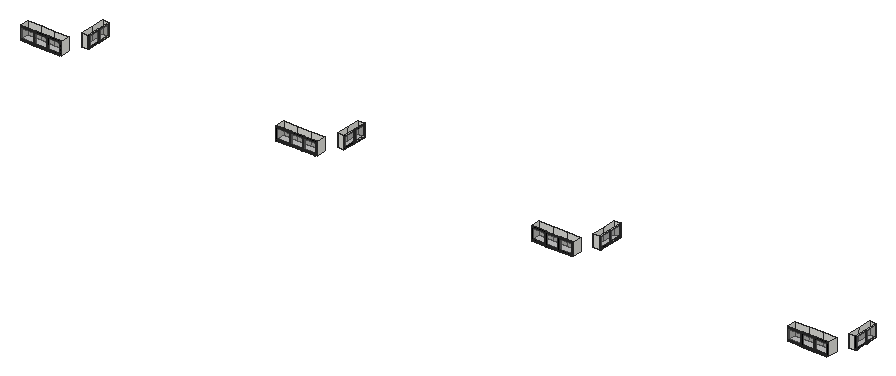
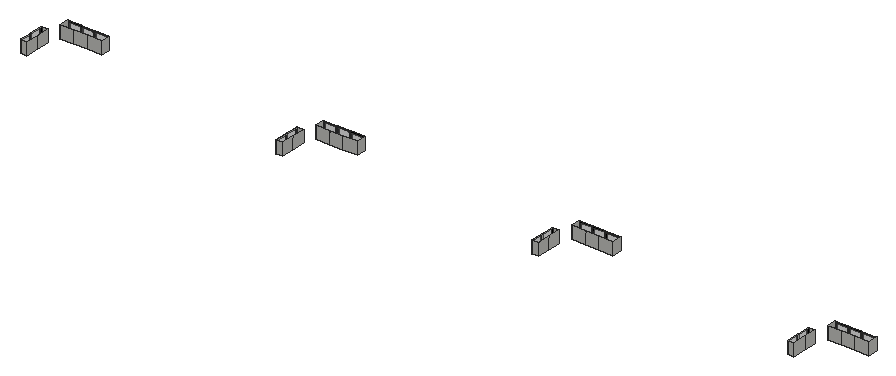
# SketchUp Ruby script. Lengths in inches.
U = 1.inch
M = Sketchup.active_model
def pt(a) = Geom::Point3d.new(a.map { |v| v * U })
def face(e, loops, mat)
  f = e.add_face(loops[0].map { |a| pt(a) })
  loops[1..].each { |l| e.add_face(l.map { |a| pt(a) }).erase! }
  f.material = f.back_material = mat if mat
  f
end
# faces: each face lists its corners as indices into pts; further lists are holes
def faces(e, pts, list, mat = nil) = list.each { |f| face(e, (f[0].is_a?(Array) ? f : [f]).map { |l| l.map { |i| pts[i] } }, mat) }
# xy, xz, yz: faces in a plane at the given z, y or x. An outline is a flat list of corners, or four numbers for a rectangle; further outlines are holes
def ring(l) = l.size == 4 ? [[l[0], l[1]], [l[2], l[1]], [l[2], l[3]], [l[0], l[3]]] : l.each_slice(2).to_a
def flat(e, list, mat, &to3) = list.each { |f| face(e, (f[0].is_a?(Array) ? f : [f]).map { |l| ring(l).map { |u, v| to3.(u, v) } }, mat) }
def xy(e, z, list, mat = nil) = flat(e, list, mat) { |x, y| [x, y, z] }
def xz(e, y, list, mat = nil) = flat(e, list, mat) { |x, z| [x, y, z] }
def yz(e, x, list, mat = nil) = flat(e, list, mat) { |y, z| [x, y, z] }
def lines(e, pts, list) = list.each { |a, b| e.add_line(pt(pts[a]), pt(pts[b])) }
# prism: a flat outline (further loops are holes) pulled along v
def prism(e, loops, v, mat = nil)
  f = face(e, loops, mat); d = Geom::Vector3d.new(v.map { |x| x * U })
  f.pushpull(f.normal.samedirection?(d) ? d.length : -d.length)
end
def box(e, o, s, mat = nil) = prism(e, [[o, [o[0] + s[0], o[1], o[2]], [o[0] + s[0], o[1] + s[1], o[2]], [o[0], o[1] + s[1], o[2]]]], [0, 0, s[2]], mat)
def at(x, y, z, deg = 0) = Geom::Transformation.translation(pt([x, y, z])) * Geom::Transformation.rotation(ORIGIN, Z_AXIS, deg.degrees)
def axes(o, x, y, z) = Geom::Transformation.new([*x, 0, *y, 0, *z, 0, *pt(o).to_a, 1])
def part(name) = M.definitions.add(name)
# library, detail: a bought-in or finely detailed component or shape, given as its bounding box
def library(name, o, s) = part(name).tap { |d| box(d.entities, o, s) }
def detail(e, o, s) = box(e.add_group.entities, o, s)
def put(e, d, t, mat = nil) = e.add_instance(d, t).tap { |i| i.material = mat if mat }
def group(e, t, mat = nil) = e.add_group.tap { |g| g.transformation = t; g.material = mat if mat }.entities
root = M.entities
M.materials.add("[Color M09]").color = [0, 0, 0]
M.materials.add("[Translucent Glass Gray]").color = [128, 128, 128]
M.materials["[Translucent Glass Gray]"].alpha = 0.5
xy(root,89.9,[[400.71,509.7,430.93,511.2],[433.56,509.7,461.15,511.2],[463.98,509.7,491.36,511.2],[990.53,509.7,1020.74,511.2],[1023.37,509.7,1050.96,511.2],
  [1053.79,509.7,1081.17,511.2],[1580.34,509.7,1610.56,511.2],[1613.18,509.7,1640.77,511.2],[1643.6,509.7,1670.99,511.2],[2170.15,509.7,2200.37,511.2],
  [2202.99,509.7,2230.58,511.2],[2233.42,509.7,2260.8,511.2],[400.71,511.2,430.93,512.7],[433.56,511.2,461.15,512.7],[463.98,511.2,491.36,512.7],
  [990.53,511.2,1020.74,512.7],[1023.37,511.2,1050.96,512.7],[1053.79,511.2,1081.17,512.7],[1580.34,511.2,1610.56,512.7],[1613.18,511.2,1640.77,512.7],
  [1643.6,511.2,1670.99,512.7],[2170.15,511.2,2200.37,512.7],[2202.99,511.2,2230.58,512.7],[2233.42,511.2,2260.8,512.7],[516.04,562.12,517.04,589.16],
  [517.04,562.12,518.04,589.16],[1105.85,562.12,1106.85,589.16],[1106.85,562.12,1107.85,589.16],[1695.66,562.12,1696.66,589.16],[1696.66,562.12,1697.66,589.16],
  [2285.48,562.12,2286.48,589.16],[2286.48,562.12,2287.48,589.16],[516.04,591.16,517.04,618.2],[517.04,591.16,518.04,618.2],[1105.85,591.16,1106.85,618.2],
  [1106.85,591.16,1107.85,618.2],[1695.66,591.16,1696.66,618.2],[1696.66,591.16,1697.66,618.2],[2285.48,591.16,2286.48,618.2],[2286.48,591.16,2287.48,618.2]],"[Color M09]")
xy(root,92.58,[[400.71,509.7,430.93,511.2],[433.56,509.7,461.15,511.2],[463.98,509.7,491.36,511.2],[990.53,509.7,1020.74,511.2],[1023.37,509.7,1050.96,511.2],
  [1053.79,509.7,1081.17,511.2],[1580.34,509.7,1610.56,511.2],[1613.18,509.7,1640.77,511.2],[1643.6,509.7,1670.99,511.2],[2170.15,509.7,2200.37,511.2],
  [2202.99,509.7,2230.58,511.2],[2233.42,509.7,2260.8,511.2],[400.71,511.2,430.93,512.7],[433.56,511.2,461.15,512.7],[463.98,511.2,491.36,512.7],
  [990.53,511.2,1020.74,512.7],[1023.37,511.2,1050.96,512.7],[1053.79,511.2,1081.17,512.7],[1580.34,511.2,1610.56,512.7],[1613.18,511.2,1640.77,512.7],
  [1643.6,511.2,1670.99,512.7],[2170.15,511.2,2200.37,512.7],[2202.99,511.2,2230.58,512.7],[2233.42,511.2,2260.8,512.7],[516.04,562.12,517.04,589.16],
  [517.04,562.12,518.04,589.16],[1105.85,562.12,1106.85,589.16],[1106.85,562.12,1107.85,589.16],[1695.66,562.12,1696.66,589.16],[1696.66,562.12,1697.66,589.16],
  [2285.48,562.12,2286.48,589.16],[2286.48,562.12,2287.48,589.16],[516.04,591.16,517.04,618.2],[517.04,591.16,518.04,618.2],[1105.85,591.16,1106.85,618.2],
  [1106.85,591.16,1107.85,618.2],[1695.66,591.16,1696.66,618.2],[1696.66,591.16,1697.66,618.2],[2285.48,591.16,2286.48,618.2],[2286.48,591.16,2287.48,618.2]],"[Color M09]")
xy(root,116.1875,[[400.71,509.7,430.93,511.2],[433.56,509.7,461.15,511.2],[463.98,509.7,491.36,511.2],[990.53,509.7,1020.74,511.2],[1023.37,509.7,1050.96,511.2],
  [1053.79,509.7,1081.17,511.2],[1580.34,509.7,1610.56,511.2],[1613.18,509.7,1640.77,511.2],[1643.6,509.7,1670.99,511.2],[2170.15,509.7,2200.37,511.2],
  [2202.99,509.7,2230.58,511.2],[2233.42,509.7,2260.8,511.2],[400.71,511.2,430.93,512.7],[433.56,511.2,461.15,512.7],[463.98,511.2,491.36,512.7],
  [990.53,511.2,1020.74,512.7],[1023.37,511.2,1050.96,512.7],[1053.79,511.2,1081.17,512.7],[1580.34,511.2,1610.56,512.7],[1613.18,511.2,1640.77,512.7],
  [1643.6,511.2,1670.99,512.7],[2170.15,511.2,2200.37,512.7],[2202.99,511.2,2230.58,512.7],[2233.42,511.2,2260.8,512.7],[516.04,562.12,517.04,589.16],
  [517.04,562.12,518.04,589.16],[1105.85,562.12,1106.85,589.16],[1106.85,562.12,1107.85,589.16],[1695.66,562.12,1696.66,589.16],[1696.66,562.12,1697.66,589.16],
  [2285.48,562.12,2286.48,589.16],[2286.48,562.12,2287.48,589.16],[516.04,591.16,517.04,618.2],[517.04,591.16,518.04,618.2],[1105.85,591.16,1106.85,618.2],
  [1106.85,591.16,1107.85,618.2],[1695.66,591.16,1696.66,618.2],[1696.66,591.16,1697.66,618.2],[2285.48,591.16,2286.48,618.2],[2286.48,591.16,2287.48,618.2]],"[Color M09]")
xz(root,511.2,[[400.71,92.58,430.93,116.1875],[433.56,92.58,461.15,116.1875],[463.98,92.58,491.36,116.1875],[990.53,92.58,1020.74,116.1875],[1023.37,92.58,1050.96,116.1875],
  [1053.79,92.58,1081.17,116.1875],[1580.34,92.58,1610.56,116.1875],[1613.18,92.58,1640.77,116.1875],[1643.6,92.58,1670.99,116.1875],[2170.15,92.58,2200.37,116.1875],
  [2202.99,92.58,2230.58,116.1875],[2233.42,92.58,2260.8,116.1875]],"[Translucent Glass Gray]")
xz(root,512.7,[[398.04,89.9,430.93,92.58],[430.93,89.9,461.15,92.58],[461.15,89.9,494.04,92.58],[987.85,89.9,1020.74,92.58],[1020.74,89.9,1050.96,92.58],
  [1050.96,89.9,1083.85,92.58],[1577.66,89.9,1610.56,92.58],[1610.56,89.9,1640.77,92.58],[1640.77,89.9,1673.66,92.58],[2167.48,89.9,2200.37,92.58],
  [2200.37,89.9,2230.58,92.58],[2230.58,89.9,2263.48,92.58],[398.04,92.58,400.71,118.87],[430.93,92.58,433.56,118.87],[461.15,92.58,463.98,118.87],
  [491.36,92.58,494.04,118.87],[987.85,92.58,990.53,118.87],[1020.74,92.58,1023.37,118.87],[1050.96,92.58,1053.79,118.87],[1081.17,92.58,1083.85,118.87],
  [1577.66,92.58,1580.34,118.87],[1610.56,92.58,1613.18,118.87],[1640.77,92.58,1643.6,118.87],[1670.99,92.58,1673.66,118.87],[2167.48,92.58,2170.15,118.87],
  [2200.37,92.58,2202.99,118.87],[2230.58,92.58,2233.42,118.87],[2260.8,92.58,2263.48,118.87],[400.71,116.1875,430.93,118.87],[433.56,116.1875,461.15,118.87],
  [463.98,116.1875,491.36,118.87],[990.53,116.1875,1020.74,118.87],[1023.37,116.1875,1050.96,118.87],[1053.79,116.1875,1081.17,118.87],[1580.34,116.1875,1610.56,118.87],
  [1613.18,116.1875,1640.77,118.87],[1643.6,116.1875,1670.99,118.87],[2170.15,116.1875,2200.37,118.87],[2202.99,116.1875,2230.58,118.87],[2233.42,116.1875,2260.8,118.87]],"[Color M09]")
xz(root,533.7,[[398.04,89.9,430.93,118.87],[430.93,89.9,461.15,118.87],[461.15,89.9,494.04,118.87],[987.85,89.9,1020.74,118.87],[1020.74,89.9,1050.96,118.87],
  [1050.96,89.9,1083.85,118.87],[1577.66,89.9,1610.56,118.87],[1610.56,89.9,1640.77,118.87],[1640.77,89.9,1673.66,118.87],[2167.48,89.9,2200.37,118.87],
  [2200.37,89.9,2230.58,118.87],[2230.58,89.9,2263.48,118.87]])
xz(root,560.12,[[501.6,89.9,516.04,118.1875],[1091.41,89.9,1105.85,118.1875],[1681.23,89.9,1695.66,118.1875],[2271.04,89.9,2285.48,118.1875]])
xz(root,562.12,[[516.04,92.58,517.04,116.1875],[517.04,92.58,518.04,116.1875],[1105.85,92.58,1106.85,116.1875],[1106.85,92.58,1107.85,116.1875],[1695.66,92.58,1696.66,116.1875],
  [1696.66,92.58,1697.66,116.1875],[2285.48,92.58,2286.48,116.1875],[2286.48,92.58,2287.48,116.1875]],"[Color M09]")
xz(root,589.16,[[516.04,92.58,517.04,116.1875],[517.04,92.58,518.04,116.1875],[1105.85,92.58,1106.85,116.1875],[1106.85,92.58,1107.85,116.1875],[1695.66,92.58,1696.66,116.1875],
  [1696.66,92.58,1697.66,116.1875],[2285.48,92.58,2286.48,116.1875],[2286.48,92.58,2287.48,116.1875]],"[Color M09]")
xz(root,591.16,[[516.04,92.58,517.04,116.1875],[517.04,92.58,518.04,116.1875],[1105.85,92.58,1106.85,116.1875],[1106.85,92.58,1107.85,116.1875],[1695.66,92.58,1696.66,116.1875],
  [1696.66,92.58,1697.66,116.1875],[2285.48,92.58,2286.48,116.1875],[2286.48,92.58,2287.48,116.1875]],"[Color M09]")
xz(root,618.2,[[516.04,92.58,517.04,116.1875],[517.04,92.58,518.04,116.1875],[1105.85,92.58,1106.85,116.1875],[1106.85,92.58,1107.85,116.1875],[1695.66,92.58,1696.66,116.1875],
  [1696.66,92.58,1697.66,116.1875],[2285.48,92.58,2286.48,116.1875],[2286.48,92.58,2287.48,116.1875]],"[Color M09]")
xz(root,620.2,[[501.6,89.9,516.04,118.1875],[1091.41,89.9,1105.85,118.1875],[1681.23,89.9,1695.66,118.1875],[2271.04,89.9,2285.48,118.1875]])
yz(root,398.04,[[512.7,89.9,533.7,118.87]])
yz(root,400.71,[[509.7,92.58,511.2,116.1875],[511.2,92.58,512.7,116.1875]],"[Color M09]")
yz(root,430.93,[[509.7,92.58,511.2,116.1875],[511.2,92.58,512.7,116.1875]],"[Color M09]")
yz(root,433.56,[[509.7,92.58,511.2,116.1875],[511.2,92.58,512.7,116.1875]],"[Color M09]")
yz(root,461.15,[[509.7,92.58,511.2,116.1875],[511.2,92.58,512.7,116.1875]],"[Color M09]")
yz(root,463.98,[[509.7,92.58,511.2,116.1875],[511.2,92.58,512.7,116.1875]],"[Color M09]")
yz(root,491.36,[[509.7,92.58,511.2,116.1875],[511.2,92.58,512.7,116.1875]],"[Color M09]")
yz(root,494.04,[[512.7,89.9,533.7,118.87]])
yz(root,501.6,[[560.12,89.9,589.16,118.1875],[589.16,89.9,620.2,118.1875]])
yz(root,516.04,[[589.16,89.9,620.2,92.58],[589.16,92.58,591.16,118.1875],[618.2,92.58,620.2,118.1875],[562.12,116.1875,589.16,118.1875],[591.16,116.1875,618.2,118.1875]])
yz(root,516.04,[[560.12,89.9,589.16,92.58],[560.12,92.58,562.12,118.1875]],"[Color M09]")
yz(root,517.04,[[562.12,92.58,589.16,116.1875],[591.16,92.58,618.2,116.1875]],"[Translucent Glass Gray]")
yz(root,987.85,[[512.7,89.9,533.7,118.87]])
yz(root,990.53,[[509.7,92.58,511.2,116.1875],[511.2,92.58,512.7,116.1875]],"[Color M09]")
yz(root,1020.74,[[509.7,92.58,511.2,116.1875],[511.2,92.58,512.7,116.1875]],"[Color M09]")
yz(root,1023.37,[[509.7,92.58,511.2,116.1875],[511.2,92.58,512.7,116.1875]],"[Color M09]")
yz(root,1050.96,[[509.7,92.58,511.2,116.1875],[511.2,92.58,512.7,116.1875]],"[Color M09]")
yz(root,1053.79,[[509.7,92.58,511.2,116.1875],[511.2,92.58,512.7,116.1875]],"[Color M09]")
yz(root,1081.17,[[509.7,92.58,511.2,116.1875],[511.2,92.58,512.7,116.1875]],"[Color M09]")
yz(root,1083.85,[[512.7,89.9,533.7,118.87]])
yz(root,1091.41,[[560.12,89.9,589.16,118.1875],[589.16,89.9,620.2,118.1875]])
yz(root,1105.85,[[589.16,89.9,620.2,92.58],[589.16,92.58,591.16,118.1875],[618.2,92.58,620.2,118.1875],[562.12,116.1875,589.16,118.1875],[591.16,116.1875,618.2,118.1875]])
yz(root,1105.85,[[560.12,89.9,589.16,92.58],[560.12,92.58,562.12,118.1875]],"[Color M09]")
yz(root,1106.85,[[562.12,92.58,589.16,116.1875],[591.16,92.58,618.2,116.1875]],"[Translucent Glass Gray]")
yz(root,1577.66,[[512.7,89.9,533.7,118.87]])
yz(root,1580.34,[[509.7,92.58,511.2,116.1875],[511.2,92.58,512.7,116.1875]],"[Color M09]")
yz(root,1610.56,[[509.7,92.58,511.2,116.1875],[511.2,92.58,512.7,116.1875]],"[Color M09]")
yz(root,1613.18,[[509.7,92.58,511.2,116.1875],[511.2,92.58,512.7,116.1875]],"[Color M09]")
yz(root,1640.77,[[509.7,92.58,511.2,116.1875],[511.2,92.58,512.7,116.1875]],"[Color M09]")
yz(root,1643.6,[[509.7,92.58,511.2,116.1875],[511.2,92.58,512.7,116.1875]],"[Color M09]")
yz(root,1670.99,[[509.7,92.58,511.2,116.1875],[511.2,92.58,512.7,116.1875]],"[Color M09]")
yz(root,1673.66,[[512.7,89.9,533.7,118.87]])
yz(root,1681.23,[[560.12,89.9,589.16,118.1875],[589.16,89.9,620.2,118.1875]])
yz(root,1695.66,[[589.16,89.9,620.2,92.58],[589.16,92.58,591.16,118.1875],[618.2,92.58,620.2,118.1875],[562.12,116.1875,589.16,118.1875],[591.16,116.1875,618.2,118.1875]])
yz(root,1695.66,[[560.12,89.9,589.16,92.58],[560.12,92.58,562.12,118.1875]],"[Color M09]")
yz(root,1696.66,[[562.12,92.58,589.16,116.1875],[591.16,92.58,618.2,116.1875]],"[Translucent Glass Gray]")
yz(root,2167.48,[[512.7,89.9,533.7,118.87]])
yz(root,2170.15,[[509.7,92.58,511.2,116.1875],[511.2,92.58,512.7,116.1875]],"[Color M09]")
yz(root,2200.37,[[509.7,92.58,511.2,116.1875],[511.2,92.58,512.7,116.1875]],"[Color M09]")
yz(root,2202.99,[[509.7,92.58,511.2,116.1875],[511.2,92.58,512.7,116.1875]],"[Color M09]")
yz(root,2230.58,[[509.7,92.58,511.2,116.1875],[511.2,92.58,512.7,116.1875]],"[Color M09]")
yz(root,2233.42,[[509.7,92.58,511.2,116.1875],[511.2,92.58,512.7,116.1875]],"[Color M09]")
yz(root,2260.8,[[509.7,92.58,511.2,116.1875],[511.2,92.58,512.7,116.1875]],"[Color M09]")
yz(root,2263.48,[[512.7,89.9,533.7,118.87]])
yz(root,2271.04,[[560.12,89.9,589.16,118.1875],[589.16,89.9,620.2,118.1875]])
yz(root,2285.48,[[589.16,89.9,620.2,92.58],[589.16,92.58,591.16,118.1875],[618.2,92.58,620.2,118.1875],[562.12,116.1875,589.16,118.1875],[591.16,116.1875,618.2,118.1875]])
yz(root,2285.48,[[560.12,89.9,589.16,92.58],[560.12,92.58,562.12,118.1875]],"[Color M09]")
yz(root,2286.48,[[562.12,92.58,589.16,116.1875],[591.16,92.58,618.2,116.1875]],"[Translucent Glass Gray]")
